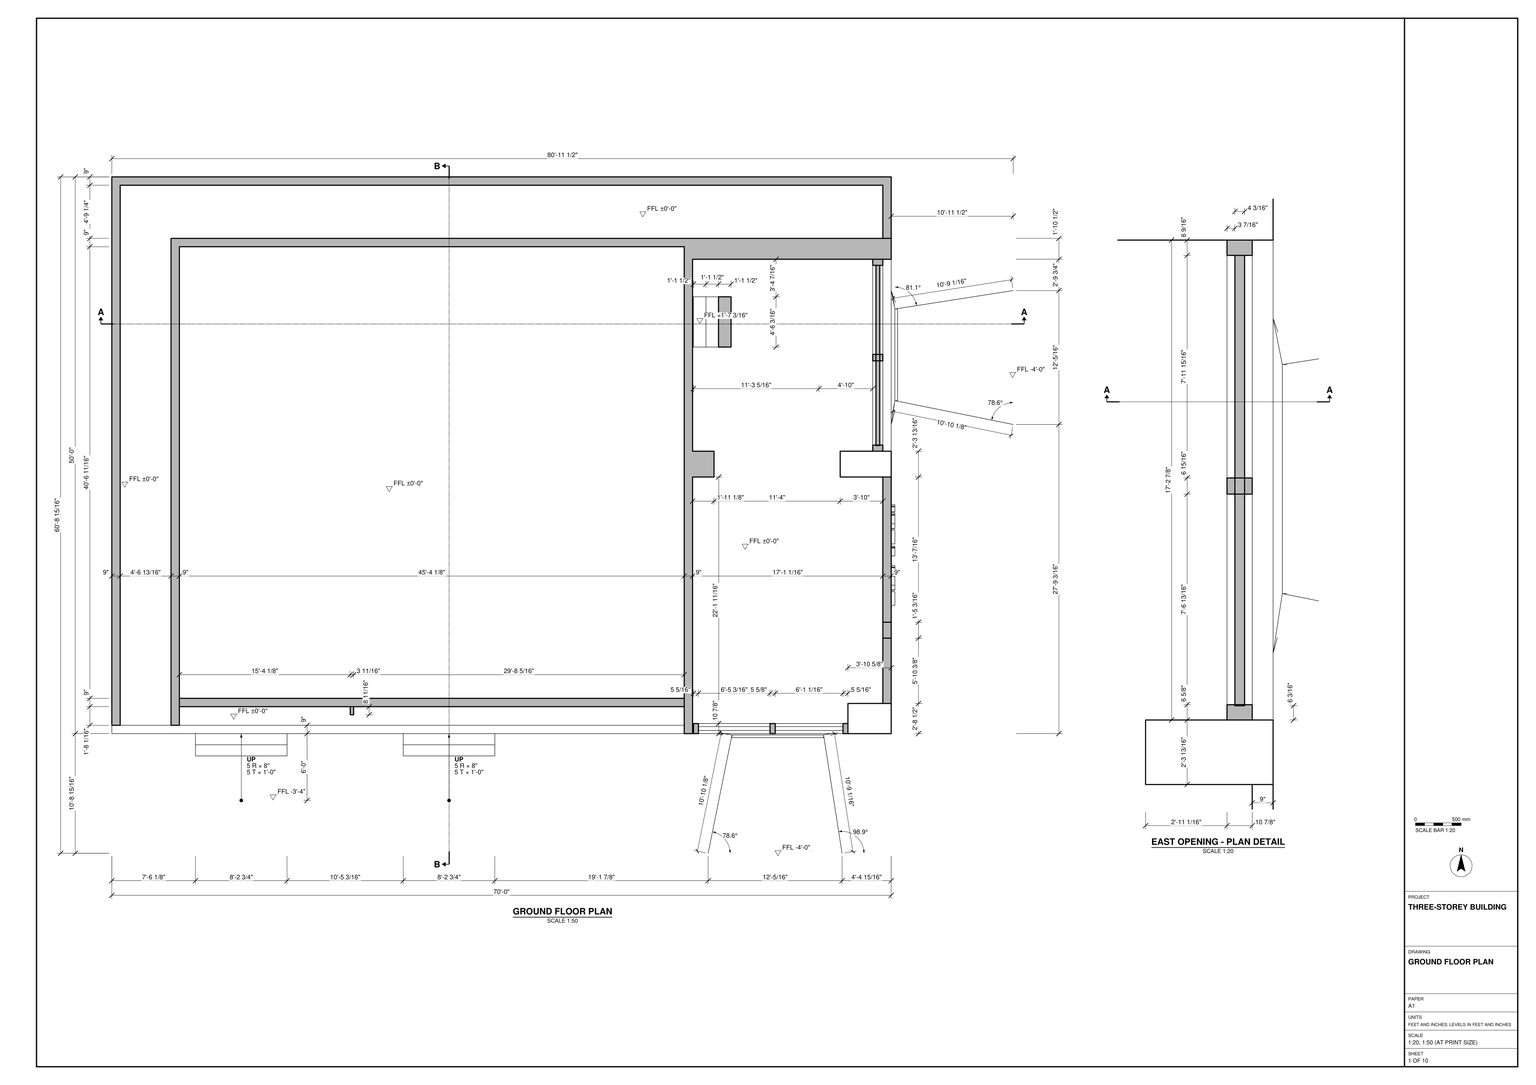
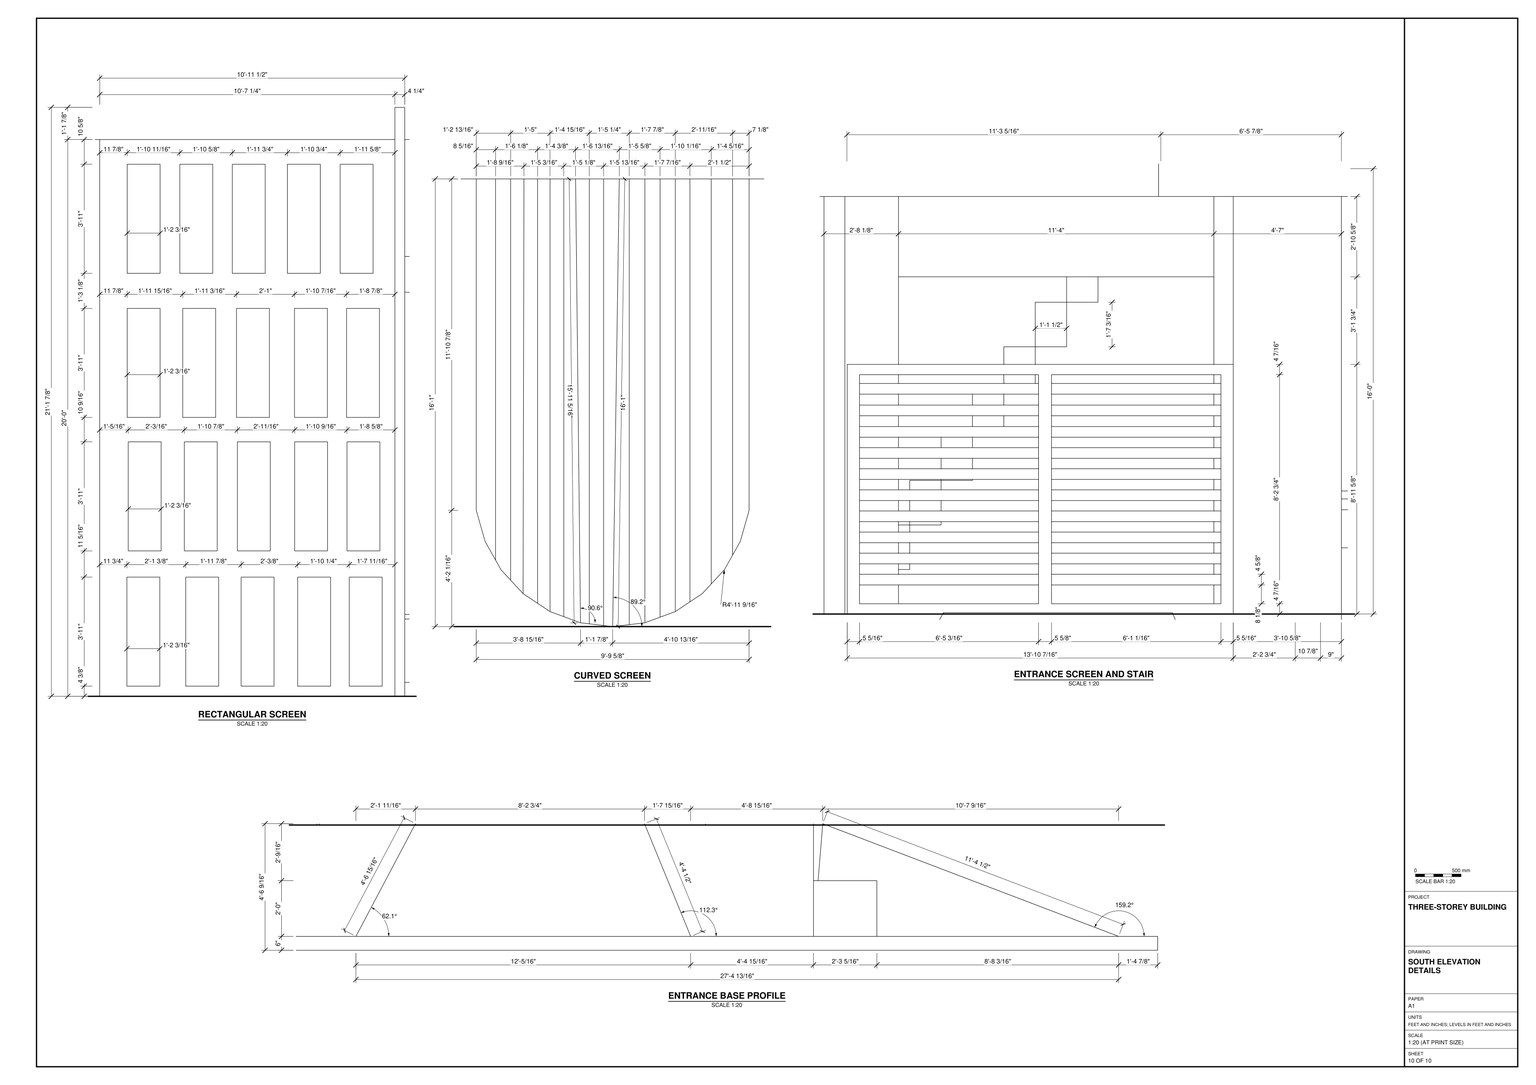
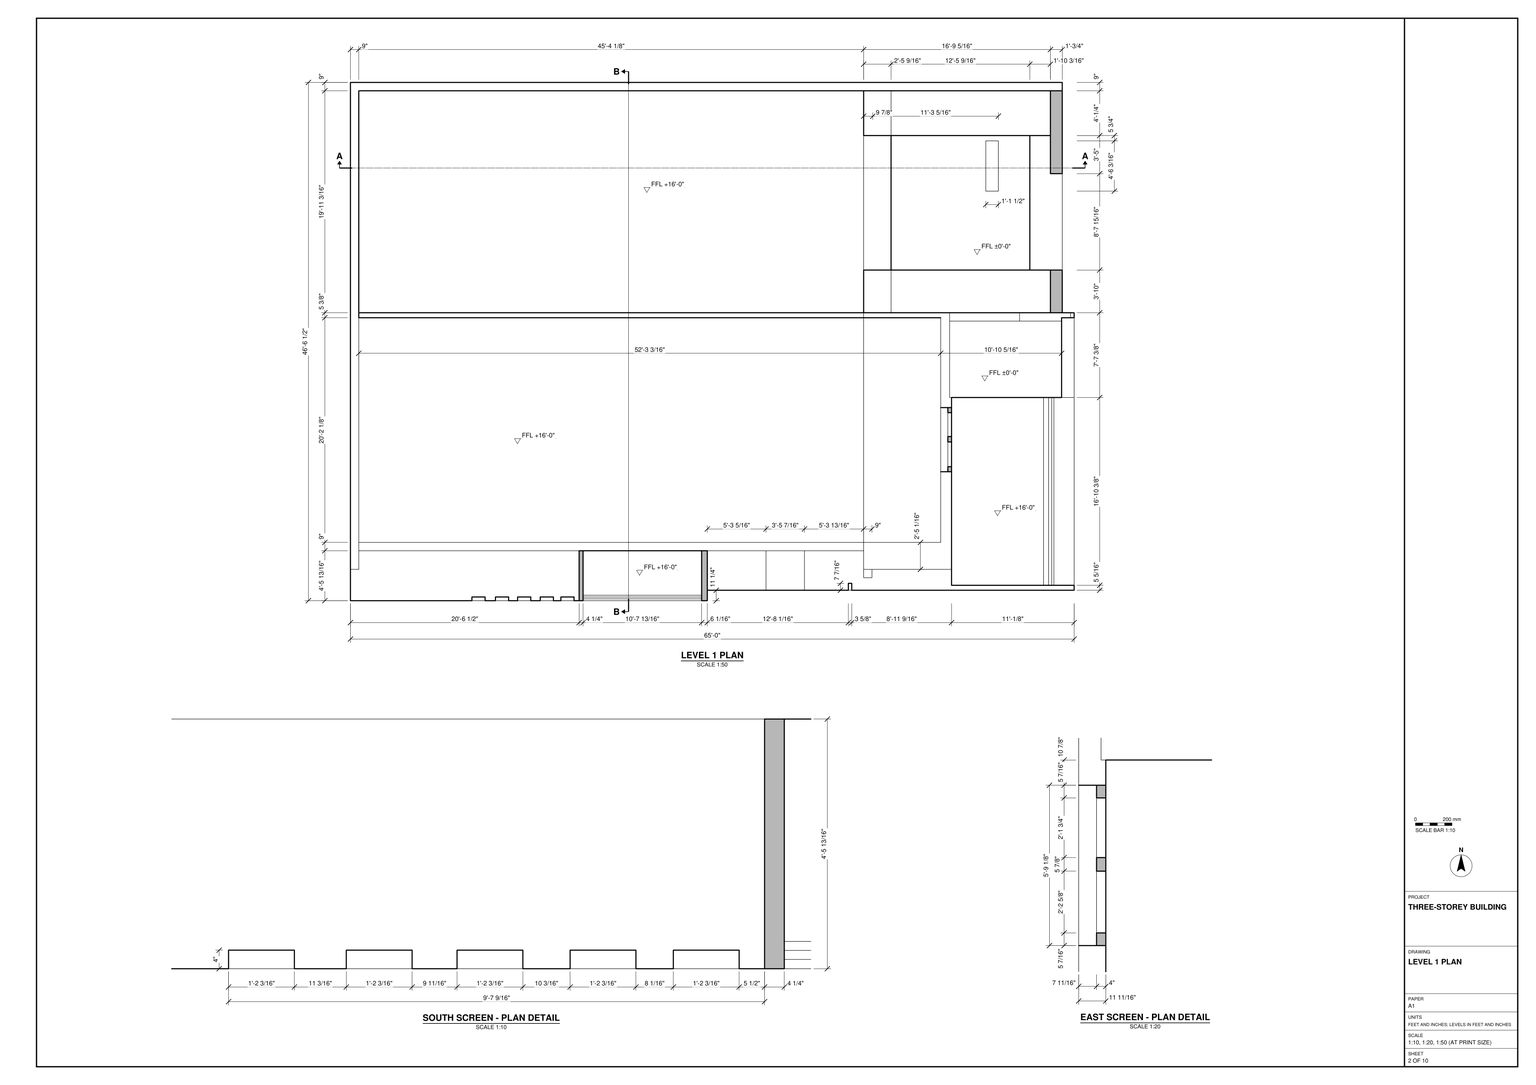
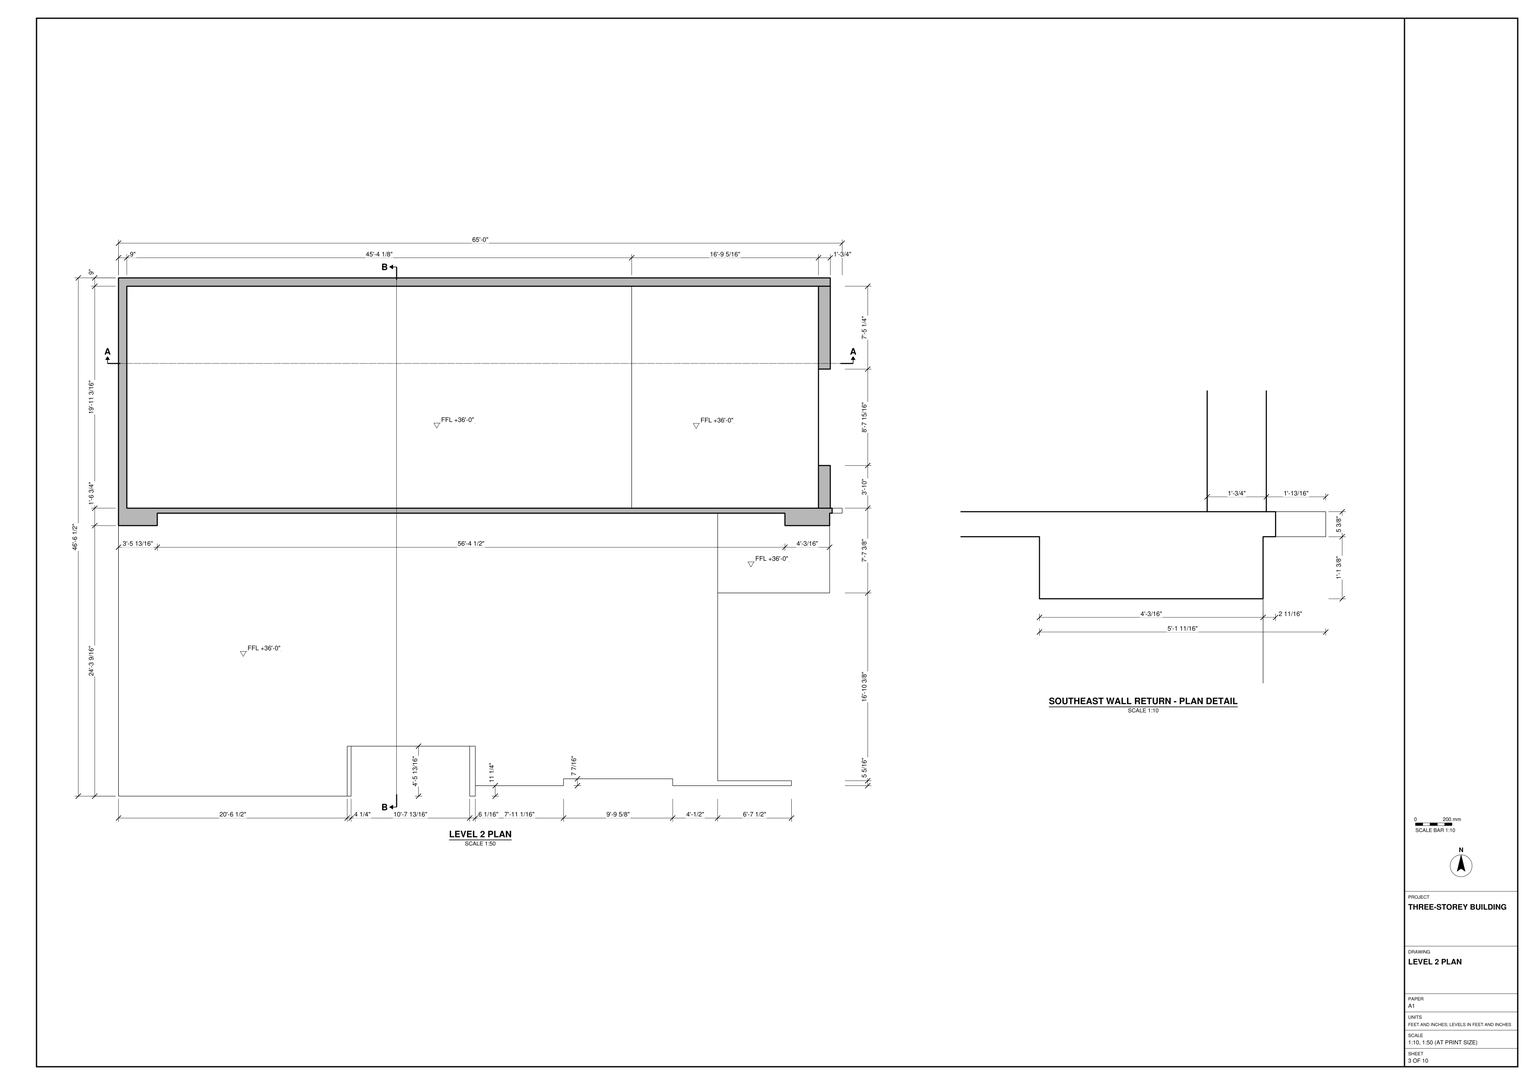
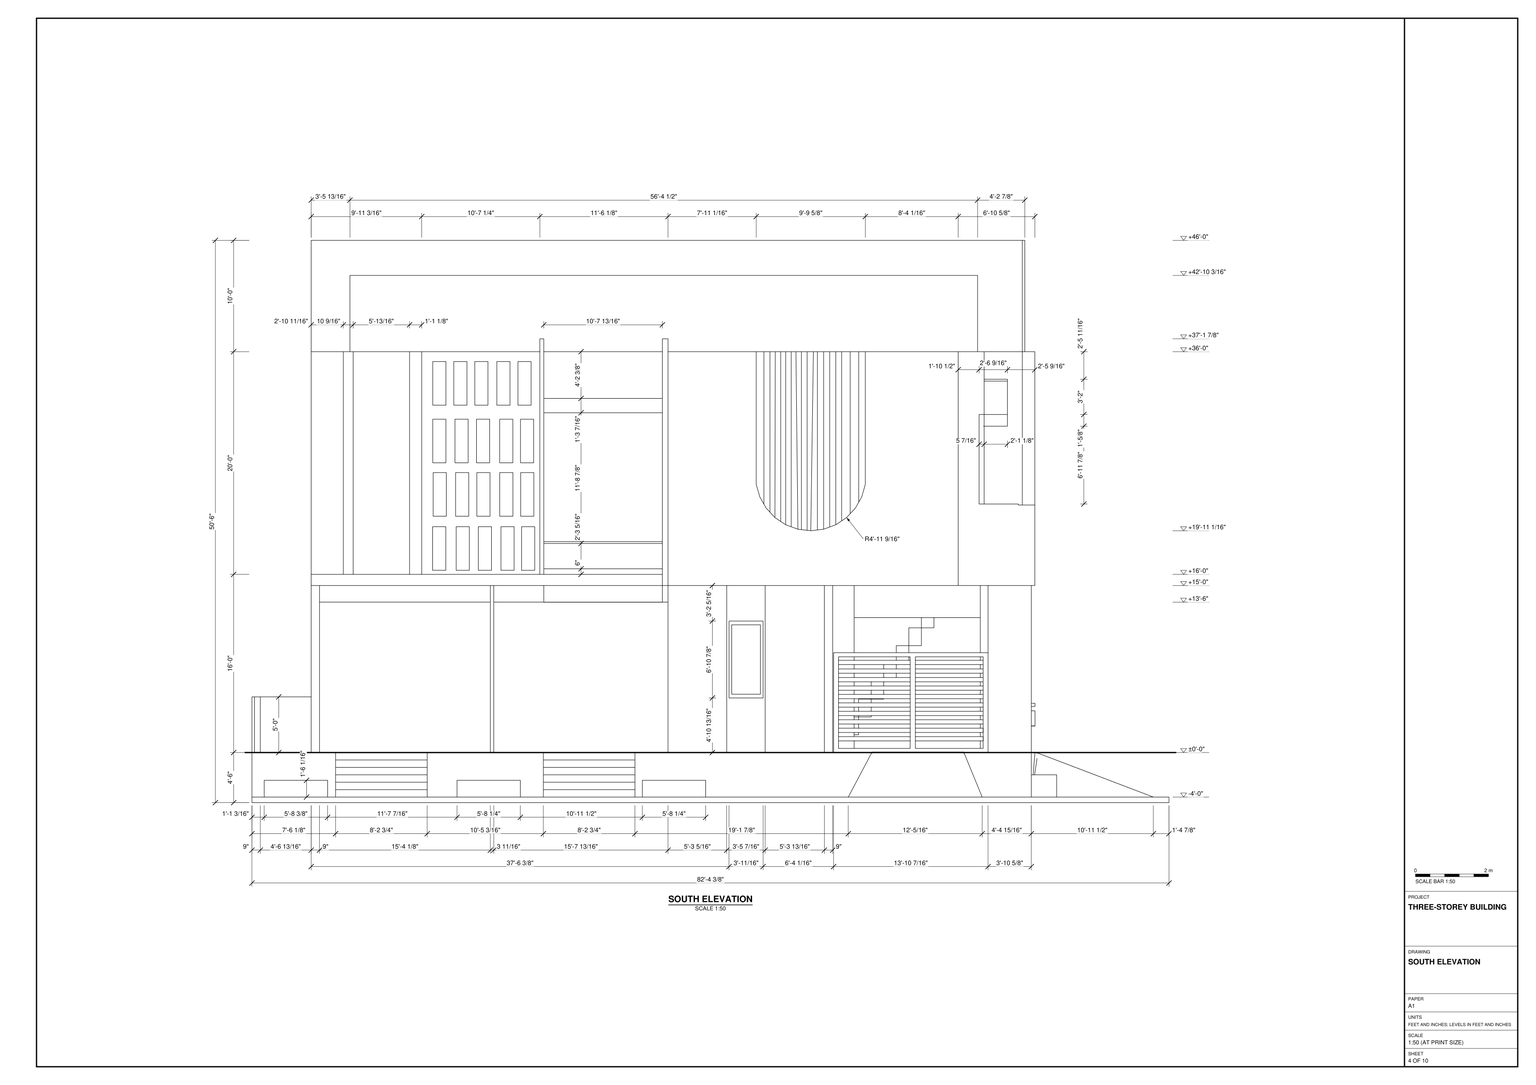
Use the plans, sections, elevations and details in task_files/diagram_01.pdf to build the three-storey building in SketchUp. Work in feet and inches. The complete model measures 82'-4 3/8" along X, 67'-10 1/8" along Y and 50'-6" along Z. Set the ground floor at ±0'-0" and the upper floors at +16'-0" and +36'-0".

Lay out the broad ground-floor space and the narrower east bay, using the wall thicknesses shown in plan. Model the floor slabs, openings, stairs and roof. Follow each floor plan rather than repeating the ground-floor outline: parts of the east bay remain open to the floor below. Include the two sets of south steps, the sloping entrance base and the framing of the east opening. Use the south elevation details to distinguish the rectangular grid screen, the vertical screen with a curved lower edge and the horizontal slats in front of the entrance stair.

Keep walls, slabs and roof as separate groups or components, and do the same for each furniture or built-in joinery piece shown. Use components for repeated parts. Any decor or loose items shown may use suitable library components. Save one SketchUp model as output_files/three_storey_building_with_facade_screens.skp.

# SketchUp Ruby script. Lengths in inches.
U = 1.inch
M = Sketchup.active_model
def pt(a) = Geom::Point3d.new(a.map { |v| v * U })
def face(e, loops, mat)
  f = e.add_face(loops[0].map { |a| pt(a) })
  loops[1..].each { |l| e.add_face(l.map { |a| pt(a) }).erase! }
  f.material = f.back_material = mat if mat
  f
end
# faces: each face lists its corners as indices into pts; further lists are holes
def faces(e, pts, list, mat = nil) = list.each { |f| face(e, (f[0].is_a?(Array) ? f : [f]).map { |l| l.map { |i| pts[i] } }, mat) }
# xy, xz, yz: faces in a plane at the given z, y or x. An outline is a flat list of corners, or four numbers for a rectangle; further outlines are holes
def ring(l) = l.size == 4 ? [[l[0], l[1]], [l[2], l[1]], [l[2], l[3]], [l[0], l[3]]] : l.each_slice(2).to_a
def flat(e, list, mat, &to3) = list.each { |f| face(e, (f[0].is_a?(Array) ? f : [f]).map { |l| ring(l).map { |u, v| to3.(u, v) } }, mat) }
def xy(e, z, list, mat = nil) = flat(e, list, mat) { |x, y| [x, y, z] }
def xz(e, y, list, mat = nil) = flat(e, list, mat) { |x, z| [x, y, z] }
def yz(e, x, list, mat = nil) = flat(e, list, mat) { |y, z| [x, y, z] }
def lines(e, pts, list) = list.each { |a, b| e.add_line(pt(pts[a]), pt(pts[b])) }
# prism: a flat outline (further loops are holes) pulled along v
def prism(e, loops, v, mat = nil)
  f = face(e, loops, mat); d = Geom::Vector3d.new(v.map { |x| x * U })
  f.pushpull(f.normal.samedirection?(d) ? d.length : -d.length)
end
def box(e, o, s, mat = nil) = prism(e, [[o, [o[0] + s[0], o[1], o[2]], [o[0] + s[0], o[1] + s[1], o[2]], [o[0], o[1] + s[1], o[2]]]], [0, 0, s[2]], mat)
def at(x, y, z, deg = 0) = Geom::Transformation.translation(pt([x, y, z])) * Geom::Transformation.rotation(ORIGIN, Z_AXIS, deg.degrees)
def axes(o, x, y, z) = Geom::Transformation.new([*x, 0, *y, 0, *z, 0, *pt(o).to_a, 1])
def part(name) = M.definitions.add(name)
# library, detail: a bought-in or finely detailed component or shape, given as its bounding box
def library(name, o, s) = part(name).tap { |d| box(d.entities, o, s) }
def detail(e, o, s) = box(e.add_group.entities, o, s)
def put(e, d, t, mat = nil) = e.add_instance(d, t).tap { |i| i.material = mat if mat }
def group(e, t, mat = nil) = e.add_group.tap { |g| g.transformation = t; g.material = mat if mat }.entities
root = M.entities
M.materials.add("[Blinds Roman Hobbled Blue]").color = [81, 82, 87]
M.materials.add("[Color C06]").color = [204, 102, 0]
M.materials.add("[Color C08]").color = [85, 51, 15]
M.materials.add("[Color D01]").color = [255, 242, 204]
M.materials.add("[Color M03]").color = [170, 170, 170]
M.materials.add("[Color M05]").color = [114, 114, 114]
M.materials.add("[Color M06]").color = [86, 86, 86]
M.materials.add("[Color M07]").color = [58, 58, 58]
M.materials.add("[Grass Dark Green]").color = [106, 157, 55]
M.materials.add("[Metal Seamed]").color = [118, 119, 115]
M.materials.add("[Rough Square Concrete Block]").color = [123, 120, 113]
M.materials.add("[Translucent Glass Blue]").color = [100, 149, 237]
M.materials["[Translucent Glass Blue]"].alpha = 0.5
M.materials.add("[Translucent Glass Gray]").color = [128, 128, 128]
M.materials["[Translucent Glass Gray]"].alpha = 0.5
c1 = library("om soni",[1.17,0,0],[108.57,24.51,4])
c2 = part("Group\#1")
xy(c2.entities,0,[[0,0,144.33,198.39]])
p = [[0,0,0],[144.33,0,0],[124.43,192.38,36.8],[25.68,192.38,36.8],[0,198.39,0],[144.33,198.39,0],
  [25.68,187.9375,35.5625],[124.43,187.9375,35.5625]]
faces(c2.entities,p,[[0,1,2,3],[0,3,4],[1,5,2],[4,6,7,5],[6,4,3],[7,2,5],[3,2,7,6]])
c3 = part("Group\#2")
box(c3.entities,[0,0,0],[20.5,54.1875,8])
c4 = library("Group\#4",[0,0,0],[166.4375,10.875,128.625])
c5 = part("Group\#5")
xy(c5.entities,0,[[0,0,18.6875,4]],"[Color C08]")
xy(c5.entities,1.47,[[1.47,0,8.67,4],[10.26,0,17.21,4]],"[Color C08]")
xy(c5.entities,28.76,[[1.47,0,8.67,4],[10.26,0,17.21,4]],"[Color C08]")
xy(c5.entities,30.24,[[0,0,18.6875,4]],"[Color C08]")
xz(c5.entities,0,[[[0,0,18.6875,30.24],[1.47,1.47,8.67,28.76],[10.26,1.47,17.21,28.76]]],"[Color C08]")
xz(c5.entities,0,[[1.47,1.47,8.67,28.76],[10.26,1.47,17.21,28.76]],"[Translucent Glass Gray]")
xz(c5.entities,4,[[[0,0,18.6875,30.24],[1.47,1.47,8.67,28.76],[10.26,1.47,17.21,28.76]]],"[Color C08]")
yz(c5.entities,0,[[0,0,4,30.24]],"[Color C08]")
yz(c5.entities,1.47,[[0,1.47,4,28.76]],"[Color C08]")
yz(c5.entities,8.67,[[0,1.47,4,28.76]],"[Color C08]")
yz(c5.entities,10.26,[[0,1.47,4,28.76]],"[Color C08]")
yz(c5.entities,17.21,[[0,1.47,4,28.76]],"[Color C08]")
yz(c5.entities,18.6875,[[0,0,4,30.24]],"[Color C08]")
xy(root,0,[[0,0,988.375,814.125]])
xy(root,6,[[90.14,142.125,188.89,154.125],[314.08,142.125,412.83,154.125],[90.14,154.125,188.89,214.125],[314.08,154.125,412.83,214.125],[0,214.125,0,814.125,840,814.125,840,521.03,867.3125,521.03,867.3125,334.22,840,334.22,840,214.125]])
xy(root,6,[[0,0,988.375,0,988.375,814.125,840,814.125,840,521.03,867.3125,521.03,867.3125,334.22,840,334.22,840,214.125,489.03,214.125,489.03,152.9375,420.78,152.9375,420.78,214.125,412.83,214.125,412.83,142.125,314.08,142.125,314.08,214.125,289.28,214.125,289.28,152.9375,221.03,152.9375,221.03,214.125,188.89,214.125,188.89,142.125,90.14,142.125,90.14,214.125,81.59,214.125,81.59,141.5625,13.22,141.5625,13.22,214.125,0,214.125]],"[Rough Square Concrete Block]")
xy(root,14,[[90.14,142.125,188.89,154.125],[314.08,142.125,412.83,154.125]])
xy(root,22,[[90.14,154.125,188.89,166.125],[314.08,154.125,412.83,166.125]])
xy(root,24.0625,[[13.22,141.5625,81.59,214.125],[221.03,152.9375,289.28,214.125],[420.78,152.9375,489.03,214.125]],"[Color C06]")
xy(root,30,[[90.14,166.125,188.89,178.125],[314.08,166.125,412.83,178.125]])
xy(root,30,[[840,334.22,867.3125,521.03]],"[Grass Dark Green]")
xy(root,38,[[90.14,178.125,188.89,190.125],[314.08,178.125,412.83,190.125]])
xy(root,46,[[90.14,190.125,188.89,202.125],[314.08,190.125,412.83,202.125]])
xy(root,54,[[90.14,202.125,188.89,214.125],[314.08,202.125,412.83,214.125],[0,214.125,616.9375,223.125],[616.9375,214.125,616.9375,738.875,72.8125,738.875,72.8125,223.125,63.8125,223.125,63.8125,747.875,840,747.875,840,725.375,625.9375,725.375,625.9375,518.5,649.05,518.5,649.05,490.6875,625.9375,490.6875,625.9375,214.125],[625.9375,214.125,793.375,223.125],
  [0,223.125,0,814.125,840,814.125,840,747.875,831,747.875,831,805.125,9,805.125,9,223.125],[9,223.125,63.8125,223.125,63.8125,747.875,831,747.875,831,805.125,9,805.125],[72.8125,223.125,616.9375,223.125,616.9375,243.1875,260.625,243.1875,260.625,234.5,256.96,234.5,256.96,243.1875,72.8125,243.1875],[625.9375,223.125,793.375,223.125,793.375,246.66,831,246.66,831,490.6875,785.03,490.6875,785.03,518.5,831,518.5,831,725.375,625.9375,725.375,625.9375,518.5,649.05,518.5,649.05,490.6875,625.9375,490.6875],[256.96,234.5,260.625,243.1875],
  [72.8125,243.1875,616.9375,252.1875],[72.8125,252.1875,616.9375,738.875],[831,334.22,840,490.6875],[785.03,490.6875,840,518.5],[831,518.5,840,725.375]])
xy(root,112.81,[[514.22,243.1875,550.9,252.1875]])
xy(root,114,[[0,223.125,9,223.125,9,805.125,831,805.125,831,747.875,840,747.875,840,814.125,0,814.125]])
xy(root,123.28,[[616.9375,358.22,625.9375,418.54]])
xy(root,126,[[831,334.22,840,412.45],[831,412.45,840,490.6875]])
xy(root,126,[[831,246.66,840,317.04]],"[Color C06]")
xy(root,130.125,[[831,317.04,840,334.22]],"[Color M06]")
xy(root,195.69,[[514.22,243.1875,550.9,252.1875]])
xy(root,196.78,[[616.9375,358.22,625.9375,418.54]])
xy(root,199.375,[[818.25,499.6875,826.05,518.5],[826.05,499.6875,831,518.5],[831,499.6875,840,518.5],[818.25,690.63,831,725.375],[831,725.375,840,747.875]])
xy(root,199.375,[[649.05,490.6875,785.03,499.6875],[818.25,518.5,831,545.69],[818.25,545.69,831,690.63]],"[Color M06]")
xy(root,216,[[314.53,193.32,442.35,195.26]])
xy(root,216.11,[[72.8125,223.125,256.96,243.1875],[260.625,223.125,448.43,243.1875]])
xy(root,234,[[63.8125,189.375,256.96,223.125],[256.96,189.375,260.625,234.5],[260.625,189.375,448.43,223.125],[448.43,200.625,511.74,243.1875],[511.74,200.625,553.15,243.1875],
  [553.15,200.625,553.15,243.1875,616.9375,243.1875,616.9375,214.125,625.9375,214.125,625.9375,490.6875,843.8125,490.6875,843.8125,200.625],[72.8125,223.125,256.96,243.1875],[260.625,223.125,448.43,243.1875],[256.96,234.5,260.625,243.1875],[72.8125,243.1875,616.9375,252.1875],
  [785.03,490.6875,840,499.6875],[840,490.6875,843.8125,499.6875],[646.5,499.6875,649.05,518.5],[785.03,499.6875,818.25,518.5],[625.9375,518.5,646.5,725.375],
  [646.5,725.375,818.25,738.875]])
xy(root,236.5,[[793.375,214.125,840,246.66]])
xy(root,242,[[72.8125,252.1875,616.9375,738.875]])
xy(root,244.1875,[[830.3,408.34,843.8125,494.3]],"[Color D01]")
xy(root,246,[[63.8125,189.375,63.8125,223.125,72.8125,223.125,72.8125,243.1875,310.29,243.1875,310.29,189.375],[310.29,189.375,314.53,243.1875],[314.53,191.375,442.35,195.26],[314.53,195.26,442.35,243.1875],[711.6875,205.9375,810.86,205.9375,810.86,408.34,711.6875,408.34,711.6875,397.46,700,397.46,700,328.34,711.6875,328.34],
  [810.86,205.9375,821.99,408.34],[821.99,205.9375,843.8125,408.34],[616.9375,223.125,616.9375,252.1875,700,252.1875,700,328.34,711.6875,328.34,711.6875,223.125],[72.8125,252.1875,616.9375,494.3],[616.9375,252.1875,700,494.3],
  [700,397.46,700,494.3,616.9375,494.3,616.9375,499.6875,709.625,499.6875,709.625,408.34,711.6875,408.34,711.6875,397.46],[72.8125,494.3,616.9375,499.6875],[72.8125,499.6875,616.9375,738.875],[616.9375,499.6875,646.5,545.69],[646.5,499.6875,818.25,545.69],
  [616.9375,545.69,646.5,690.63],[616.9375,690.63,646.5,738.875],[646.5,690.63,818.25,738.875],[818.25,690.63,831,738.875]])
xy(root,246,[[314.53,189.375,442.35,191.375],[796.0625,545.69,831,545.69,831,649.6,818.25,649.6,818.25,690.63,796.0625,690.63]],"[Color M06]")
xy(root,250.375,[[194.74,189.375,208.93,193.375],[220.12,189.375,234.31,193.375],[243.99,189.375,258.18,193.375],[268.37,189.375,282.56,193.375],[290.62,189.375,304.81,193.375]])
xy(root,252,[[314.53,191.375,442.35,193.32],[314.53,193.32,442.35,195.26]])
xy(root,255,[[810.86,205.9375,816.29,408.34],[816.29,205.9375,819.67,408.34]])
xy(root,255,[[819.67,205.9375,821.99,408.34]],"[Color M05]")
xy(root,279.3125,[[314.53,193.32,442.35,195.26]])
xy(root,281.3125,[[314.53,193.32,442.35,195.26]],"[Metal Seamed]")
xy(root,289.25,[[816.29,205.9375,819.67,408.34]])
xy(root,291.25,[[816.29,205.9375,819.67,408.34]],"[Color M07]")
xy(root,297.375,[[194.74,189.375,208.93,193.375],[220.12,189.375,234.31,193.375],[243.99,189.375,258.18,193.375],[268.37,189.375,282.56,193.375],[290.62,189.375,304.81,193.375]])
xy(root,308.69,[[195.32,189.375,209.51,193.375],[219.51,189.375,233.69,193.375],[242.38,189.375,256.57,193.375],[267.07,189.375,281.26,193.375],[289.63,189.375,303.82,193.375]])
xy(root,320.74,[[826.05,200.625,843.8125,202.125],[826.05,202.125,843.8125,205.9375]])
xy(root,321.8,[[783.69,200.625,789.14,200.625,789.14,205.9375],[783.69,200.625,789.14,205.9375,783.69,205.9375],[789.14,200.625,826.05,205.9375]])
xy(root,341.6875,[[646.5,545.69,796.0625,690.63]])
xy(root,355.69,[[195.32,189.375,209.51,193.375],[219.51,189.375,233.69,193.375],[242.38,189.375,256.57,193.375],[267.07,189.375,281.26,193.375],[289.63,189.375,303.82,193.375]])
xy(root,358.5,[[700,328.34,711.6875,397.46]])
xy(root,366.22,[[194.875,189.375,209.0625,193.375],[218.8125,189.375,233,193.375],[242,189.375,256.1875,193.375],[267,189.375,281.1875,193.375],[289.4375,189.375,303.625,193.375]])
xy(root,405.69,[[711.6875,205.9375,814.25,408.34]],"[Color M05]")
xy(root,413.22,[[194.875,189.375,209.0625,193.375],[218.8125,189.375,233,193.375],[242,189.375,256.1875,193.375],[267,189.375,281.1875,193.375],[289.4375,189.375,303.625,193.375]])
xy(root,418.3,[[783.69,200.625,789.14,205.9375,789.14,200.625],[709.625,205.9375,785,205.9375,785,211.01,810.58,211.01,810.58,408.34,709.625,408.34],[785,205.9375,785,211.01,810.58,211.01,810.58,408.34,814.25,408.34,814.25,205.9375]])
xy(root,419.75,[[616.9375,545.69,796.0625,690.63],[796.0625,545.69,818.25,690.63]])
xy(root,420.16,[[314.53,198.625,442.35,243.1875]])
xy(root,428.35,[[194.875,189.375,209.0625,193.375],[217.5625,189.375,231.75,193.375],[240.1875,189.375,254.375,193.375],[263.9375,189.375,278.125,193.375],[286.6875,189.375,300.875,193.375]])
xy(root,435.62,[[314.53,198.625,442.35,243.1875]],"[Grass Dark Green]")
xy(root,454.3,[[785,205.9375,785,211.01,810.58,211.01,810.58,408.34,814.25,408.34,814.25,205.9375]])
xy(root,456.3,[[785,205.9375,814.25,205.9375,814.25,408.34,810.58,408.34,810.58,211.01,785,211.01]],"[Color M07]")
xy(root,475.35,[[194.875,189.375,209.0625,193.375],[217.5625,189.375,231.75,193.375],[240.1875,189.375,254.375,193.375],[263.9375,189.375,278.125,193.375],[286.6875,189.375,300.875,193.375]])
xy(root,486,[[63.8125,189.375,310.29,189.375,310.29,243.1875,448.43,243.1875,448.43,200.625,543.48,200.625,543.48,208.0625,661.1,208.0625,661.1,200.625,789.14,200.625,789.14,205.9375,709.625,205.9375,709.625,494.3,105.6,494.3,105.6,480.92,63.8125,480.92],[72.8125,480.92,105.6,494.3],[782.1,480.92,782.1,494.3,72.8125,494.3,72.8125,499.6875,833,499.6875,833,494.3,830.3,494.3,830.3,480.92],[72.8125,499.6875,616.9375,738.875],[616.9375,499.6875,818.25,738.875]])
xy(root,486,[[709.625,408.34,830.3,408.34,830.3,480.92,782.1,480.92,782.1,494.3,709.625,494.3]],"[Color C06]")
xy(root,486,[[833,494.3,843.8125,499.6875]],"[Color D01]")
xy(root,499.875,[[310.29,189.375,314.53,243.1875],[442.35,189.375,448.43,243.1875]],"[Color M06]")
xy(root,549.25,[[818.25,545.69,831,649.6]],"[Color M06]")
xy(root,568.1875,[[105.6,480.92,782.1,494.3]],"[Color M05]")
xy(root,606,[[72.8125,499.6875,818.25,738.875]])
xy(root,606,[[63.8125,480.92,830.3,480.92,830.3,494.3,833,494.3,833,499.6875,72.8125,499.6875,72.8125,738.875,831,738.875,831,747.875,63.8125,747.875],[818.25,499.6875,831,738.875]],"[Color M05]")
xz(root,0,[[0,0,988.375,6]])
xz(root,141.5625,[[13.22,6,81.59,24.0625]],"[Color C06]")
xz(root,142.125,[[90.14,6,188.89,14],[314.08,6,412.83,14]])
xz(root,152.9375,[[221.03,6,289.28,24.0625],[420.78,6,489.03,24.0625]],"[Color C06]")
xz(root,154.125,[[90.14,14,188.89,22],[314.08,14,412.83,22]])
xz(root,166.125,[[90.14,22,188.89,30],[314.08,22,412.83,30]])
xz(root,178.125,[[90.14,30,188.89,38],[314.08,30,412.83,38]])
xz(root,189.375,[[63.8125,246,98.49,486],[109.07,246,169.87,486],[[183.02,246,310.29,486],[194.875,428.35,209.0625,475.35],[217.5625,428.35,231.75,475.35],[240.1875,428.35,254.375,475.35],[263.9375,428.35,278.125,475.35],[286.6875,428.35,300.875,475.35],[194.875,366.22,209.0625,413.22],[218.8125,366.22,233,413.22],[242,366.22,256.1875,413.22],[267,366.22,281.1875,413.22],[289.4375,366.22,303.625,413.22],[195.32,308.69,209.51,355.69],[219.51,308.69,233.69,355.69],[242.38,308.69,256.57,355.69],[267.07,308.69,281.26,355.69],[289.63,308.69,303.82,355.69],[194.74,250.375,208.93,297.375],[220.12,250.375,234.31,297.375],[243.99,250.375,258.18,297.375],[268.37,250.375,282.56,297.375],[290.62,250.375,304.81,297.375]]])
xz(root,189.375,[[63.8125,234,442.35,246],[442.35,234,448.43,499.875],[98.49,246,109.07,486],[169.87,246,183.02,486],[310.29,246,314.53,499.875]],"[Color M06]")
xz(root,190.125,[[90.14,38,188.89,46],[314.08,38,412.83,46]])
xz(root,191.375,[[314.53,246,442.35,252]])
xz(root,193.32,[[314.53,216,442.35,252]])
xz(root,193.32,[[314.53,279.3125,442.35,281.3125]],"[Metal Seamed]")
xz(root,193.32,[[314.53,252,442.35,279.3125]],"[Translucent Glass Blue]")
xz(root,193.375,[[194.74,250.375,208.93,297.375],[220.12,250.375,234.31,297.375],[243.99,250.375,258.18,297.375],[268.37,250.375,282.56,297.375],[290.62,250.375,304.81,297.375],
  [195.32,308.69,209.51,355.69],[219.51,308.69,233.69,355.69],[242.38,308.69,256.57,355.69],[267.07,308.69,281.26,355.69],[289.63,308.69,303.82,355.69],
  [194.875,366.22,209.0625,413.22],[218.8125,366.22,233,413.22],[242,366.22,256.1875,413.22],[267,366.22,281.1875,413.22],[289.4375,366.22,303.625,413.22],
  [194.875,428.35,209.0625,475.35],[217.5625,428.35,231.75,475.35],[240.1875,428.35,254.375,475.35],[263.9375,428.35,278.125,475.35],[286.6875,428.35,300.875,475.35]])
xz(root,195.26,[[314.53,216,442.35,246],[314.53,246,442.35,252]])
xz(root,195.26,[[314.53,279.3125,442.35,281.3125]],"[Metal Seamed]")
xz(root,195.26,[[314.53,252,442.35,279.3125]],"[Translucent Glass Blue]")
xz(root,198.625,[[314.53,420.16,442.35,435.62]])
xz(root,200.625,[[448.43,234,761.19,234,761.19,486,661.1,486,661.1,343.125,657.28,329.68,650.42,317.5,640.92,307.25,629.29,299.5,616.17,294.67,602.29,293.03,588.41,294.67,575.29,299.5,563.66,307.25,554.16,317.5,547.3,329.68,543.48,343.125,543.48,486,448.43,486],[761.19,234,843.8125,234,843.8125,320.74,826.05,320.74,826.05,321.8,783.69,321.8,783.69,418.3,789.14,418.3,789.14,486,761.19,486]])
xz(root,202.125,[[90.14,46,188.89,54],[314.08,46,412.83,54]])
xz(root,205.9375,[[711.6875,246,711.6875,405.69,789.14,405.69,789.14,321.8,783.69,321.8,783.69,320.74,843.8125,320.74,843.8125,246,821.99,246,821.99,255,819.67,255,819.67,291.25,816.29,291.25,816.29,255,810.86,255,810.86,246],[810.86,246,821.99,255],[816.29,255,819.67,289.25],[816.29,289.25,819.67,291.25],[783.69,320.74,789.14,321.8],
  [789.14,320.74,826.05,321.8],[709.625,418.3,709.625,486,789.14,486,789.14,456.3,785,456.3,785,418.3],[785,418.3,789.14,454.3],[785,454.3,789.14,456.3]])
xz(root,205.9375,[[789.14,405.69,814.25,418.3]],"[Color M05]")
xz(root,205.9375,[[789.14,454.3,814.25,456.3]],"[Color M07]")
xz(root,205.9375,[[789.14,418.3,814.25,454.3]],"[Translucent Glass Gray]")
xz(root,208.0625,[[602.29,293.03,605.13,486,598.375,486,598.375,293.49],[602.29,293.03,609.44,293.875,609.44,486,605.13,486],[598.375,293.49,598.375,486,592.21,486,592.21,294.22],[609.44,293.875,616.17,294.67,616.17,486,609.44,486],[592.21,294.22,592.21,486,586.3,486,588.41,294.67],
  [588.41,294.67,586.3,486,581.22,486,581.22,297.3125],[616.17,294.67,622.73,297.08,622.73,486,616.17,486],[622.73,297.08,629.29,299.5,629.29,486,622.73,486],[581.22,297.3125,581.22,486,575.29,486,575.29,299.5],[575.29,299.5,575.29,486,569.91,486,569.91,303.09],
  [629.29,299.5,635.59,303.7,635.59,486,629.29,486],[569.91,303.09,569.91,486,564.04,486,563.66,307.25],[635.59,303.7,640.92,307.25,644.79,311.43,644.79,486,635.59,486],[563.66,307.25,564.04,486,558.3,486,558.3,313.04],[644.79,311.43,650.42,317.5,653.99,323.85,653.99,486,644.79,486],
  [558.3,313.04,558.3,486,551.79,486,551.79,321.71,554.16,317.5],[551.79,321.71,551.79,486,543.48,486,543.48,343.125,547.3,329.68],[653.99,323.85,657.28,329.68,661.1,343.125,661.1,486,653.99,486]],"[Color C06]")
xz(root,211.01,[[785,454.3,810.58,456.3]],"[Color M07]")
xz(root,211.01,[[785,418.3,810.58,454.3]],"[Translucent Glass Gray]")
xz(root,214.125,[[0,6,13.22,6,13.22,24.0625,81.59,24.0625,81.59,6,90.14,6,90.14,54,0,54],[13.22,6,81.59,24.0625],[90.14,6,188.89,10.97],[188.89,6,221.03,6,221.03,24.0625,289.28,24.0625,289.28,6,314.08,6,314.08,54,188.89,54],[221.03,6,289.28,24.0625],
  [314.08,6,412.83,46],[420.78,6,489.03,24.0625],[90.14,10.97,188.89,46],[90.14,46,188.89,54],[314.08,46,412.83,54],
  [616.9375,54,625.9375,234]])
xz(root,214.125,[[412.83,6,420.78,6,420.78,24.0625,489.03,24.0625,489.03,6,840,6,840,236.5,793.375,236.5,793.375,54,412.83,54]],"[Color M06]")
xz(root,223.125,[[0,54,2.75,114],[2.75,54,9,114],[63.8125,54,72.8125,234],[72.8125,216.11,256.96,234],[260.625,216.11,448.43,234],
  [63.8125,234,72.8125,246]])
xz(root,234.5,[[256.96,54,260.625,234]])
xz(root,243.1875,[[256.96,54,260.625,234],[448.43,54,511.74,234],[553.15,54,616.9375,234],[72.8125,216.11,256.96,234],[260.625,216.11,448.43,234],
  [72.8125,234,448.43,246],[310.29,246,314.53,486],[442.35,246,448.43,486],[314.53,420.16,442.35,435.62],[314.53,435.62,442.35,486],
  [310.29,486,314.53,499.875],[442.35,486,448.43,499.875]])
xz(root,243.1875,[[72.8125,54,256.96,216.11],[260.625,54,448.43,216.11]],"[Blinds Roman Hobbled Blue]")
xz(root,243.1875,[[[511.74,54,553.15,234],[514.22,112.81,550.9,195.69]],[314.53,246,442.35,420.16]],"[Color M06]")
xz(root,246.66,[[831,54,840,126]])
xz(root,246.66,[[793.375,54,793.375,236.5,840,236.5,840,126,831,126,831,54]],"[Color M06]")
xz(root,252.1875,[[[72.8125,54,616.9375,234],[514.22,112.81,550.9,195.69]],[72.8125,234,616.9375,242],[72.8125,242,616.9375,246]])
xz(root,317.04,[[831,54,840,126]])
xz(root,317.04,[[831,126,840,130.125]],"[Color M06]")
xz(root,328.34,[[700,246,711.6875,358.5]])
xz(root,334.22,[[831,54,840,126],[831,126,840,130.125]])
xz(root,334.22,[[840,6,867.3125,30]],"[Color M06]")
xz(root,358.22,[[616.9375,123.28,625.9375,196.78]])
xz(root,397.46,[[700,246,711.6875,358.5]])
xz(root,408.34,[[830.3,244.1875,843.8125,246],[810.86,246,821.99,255],[816.29,255,819.67,289.25],[816.29,289.25,819.67,291.25],[810.58,418.3,814.25,454.3],
  [810.58,454.3,814.25,456.3]])
xz(root,408.34,[[711.6875,246,810.86,246,810.86,255,816.29,255,816.29,291.25,819.67,291.25,819.67,255,821.99,255,821.99,246,830.3,246,830.3,486,709.625,486,709.625,418.3,810.58,418.3,810.58,456.3,814.25,456.3,814.25,405.69,711.6875,405.69]],"[Color C06]")
xz(root,418.54,[[616.9375,123.28,625.9375,196.78]])
xz(root,480.92,[[63.8125,486,105.6,486,105.6,568.1875,782.1,568.1875,782.1,486,830.3,486,830.3,606,63.8125,606]],"[Color M05]")
xz(root,490.6875,[[831,54,840,126]])
xz(root,490.6875,[[625.9375,54,649.05,234],[785.03,54,831,54,831,126,840,126,840,234,785.03,234],[649.05,199.375,785.03,234]],"[Color M06]")
xz(root,494.3,[[72.8125,246,700,486],[830.3,486,833,606]])
xz(root,494.3,[[830.3,244.1875,843.8125,486]],"[Color D01]")
xz(root,494.3,[[105.6,486,782.1,568.1875]],"[Color M05]")
xz(root,499.6875,[[818.25,199.375,826.05,234],[826.05,199.375,831,234],[831,199.375,840,234],[831,234,843.8125,246],[72.8125,246,616.9375,486],
  [616.9375,246,818.25,486],[818.25,246,831,486],[72.8125,486,616.9375,606],[616.9375,486,818.25,606],[818.25,486,831,606],
  [831,486,833,606]])
xz(root,499.6875,[[831,246,843.8125,486]],"[Color D01]")
xz(root,499.6875,[[649.05,199.375,649.05,234,646.5,234,646.5,246,818.25,246,818.25,234,785.03,234,785.03,199.375]],"[Color M06]")
xz(root,518.5,[[625.9375,54,649.05,234],[785.03,54,785.03,234,818.25,234,818.25,199.375,840,199.375,840,54]],"[Color M06]")
xz(root,521.03,[[840,6,867.3125,30]],"[Color M06]")
xz(root,545.69,[[818.25,199.375,831,246],[616.9375,246,616.9375,419.75,796.0625,419.75,796.0625,341.6875,646.5,341.6875,646.5,246],[646.5,246,796.0625,341.6875]])
xz(root,545.69,[[796.0625,246,818.25,419.75],[818.25,246,831,549.25]],"[Color M06]")
xz(root,649.6,[[818.25,246,831,549.25]],"[Color M06]")
xz(root,690.63,[[818.25,199.375,831,246],[616.9375,246,646.5,246,646.5,341.6875,796.0625,341.6875,796.0625,419.75,616.9375,419.75],[646.5,246,796.0625,341.6875],[796.0625,246,818.25,419.75]])
xz(root,725.375,[[625.9375,54,840,54,840,199.375,818.25,199.375,818.25,234,625.9375,234]],"[Color M06]")
xz(root,738.875,[[72.8125,54,616.9375,234],[72.8125,234,616.9375,242],[646.5,234,818.25,246],[72.8125,242,616.9375,246],[72.8125,246,616.9375,486],
  [616.9375,246,818.25,486],[818.25,246,831,606],[72.8125,486,88.4375,606],[88.4375,486,616.9375,606],[616.9375,486,818.25,606]])
xz(root,747.875,[[63.8125,54,63.8125,234,831,234,831,199.375,840,199.375,840,114,831,114,831,54],[831,54,840,114],[63.8125,234,831,246],[63.8125,246,831,606]])
xz(root,805.125,[[9,54,831,114]])
xz(root,814.125,[[0,0,988.375,6],[0,6,840,54],[0,54,840,114]])
yz(root,0,[[0,0,814.125,6],[214.125,6,814.125,54],[223.125,54,814.125,114]])
yz(root,9,[[223.125,54,805.125,114]])
yz(root,13.22,[[141.5625,6,214.125,24.0625]],"[Color C06]")
yz(root,63.8125,[[223.125,54,747.875,234],[189.375,234,223.125,246],[223.125,234,747.875,246],[189.375,246,189.375,486,480.92,486,480.92,606,747.875,606,747.875,246]])
yz(root,72.8125,[[223.125,54,243.1875,216.11],[243.1875,54,252.1875,234],[252.1875,54,738.875,234],[223.125,216.11,243.1875,234],[223.125,234,243.1875,246],
  [243.1875,234,252.1875,246],[252.1875,234,738.875,242],[252.1875,242,738.875,246],[494.3,246,499.6875,486],[499.6875,246,738.875,486],
  [499.6875,486,738.875,606]])
yz(root,81.59,[[141.5625,6,214.125,24.0625]],"[Color C06]")
yz(root,90.14,[[142.125,6,142.125,14,154.125,14,154.125,22,166.125,22,166.125,30,178.125,30,178.125,38,190.125,38,190.125,46,202.125,46,202.125,54,214.125,54,214.125,6]])
yz(root,105.6,[[480.92,486,494.3,568.1875]],"[Color M05]")
yz(root,188.89,[[142.125,6,214.125,6,214.125,54,202.125,54,202.125,46,190.125,46,190.125,38,178.125,38,178.125,30,166.125,30,166.125,22,154.125,22,154.125,14,142.125,14]])
yz(root,194.74,[[189.375,250.375,193.375,297.375]])
yz(root,194.875,[[189.375,366.22,193.375,413.22],[189.375,428.35,193.375,475.35]])
yz(root,195.32,[[189.375,308.69,193.375,355.69]])
yz(root,208.93,[[189.375,250.375,193.375,297.375]])
yz(root,209.0625,[[189.375,366.22,193.375,413.22],[189.375,428.35,193.375,475.35]])
yz(root,209.51,[[189.375,308.69,193.375,355.69]])
yz(root,217.5625,[[189.375,428.35,193.375,475.35]])
yz(root,218.8125,[[189.375,366.22,193.375,413.22]])
yz(root,219.51,[[189.375,308.69,193.375,355.69]])
yz(root,220.12,[[189.375,250.375,193.375,297.375]])
yz(root,221.03,[[152.9375,6,214.125,24.0625]],"[Color C06]")
yz(root,231.75,[[189.375,428.35,193.375,475.35]])
yz(root,233,[[189.375,366.22,193.375,413.22]])
yz(root,233.69,[[189.375,308.69,193.375,355.69]])
yz(root,234.31,[[189.375,250.375,193.375,297.375]])
yz(root,240.1875,[[189.375,428.35,193.375,475.35]])
yz(root,242,[[189.375,366.22,193.375,413.22]])
yz(root,242.38,[[189.375,308.69,193.375,355.69]])
yz(root,243.99,[[189.375,250.375,193.375,297.375]])
yz(root,254.375,[[189.375,428.35,193.375,475.35]])
yz(root,256.1875,[[189.375,366.22,193.375,413.22]])
yz(root,256.57,[[189.375,308.69,193.375,355.69]])
yz(root,256.96,[[234.5,54,243.1875,216.11],[223.125,216.11,234.5,234],[234.5,216.11,243.1875,234]])
yz(root,258.18,[[189.375,250.375,193.375,297.375]])
yz(root,260.625,[[234.5,54,243.1875,216.11],[223.125,216.11,234.5,234],[234.5,216.11,243.1875,234]])
yz(root,263.9375,[[189.375,428.35,193.375,475.35]])
yz(root,267,[[189.375,366.22,193.375,413.22]])
yz(root,267.07,[[189.375,308.69,193.375,355.69]])
yz(root,268.37,[[189.375,250.375,193.375,297.375]])
yz(root,278.125,[[189.375,428.35,193.375,475.35]])
yz(root,281.1875,[[189.375,366.22,193.375,413.22]])
yz(root,281.26,[[189.375,308.69,193.375,355.69]])
yz(root,282.56,[[189.375,250.375,193.375,297.375]])
yz(root,286.6875,[[189.375,428.35,193.375,475.35]])
yz(root,289.28,[[152.9375,6,214.125,24.0625]],"[Color C06]")
yz(root,289.4375,[[189.375,366.22,193.375,413.22]])
yz(root,289.63,[[189.375,308.69,193.375,355.69]])
yz(root,290.62,[[189.375,250.375,193.375,297.375]])
yz(root,300.875,[[189.375,428.35,193.375,475.35]])
yz(root,303.625,[[189.375,366.22,193.375,413.22]])
yz(root,303.82,[[189.375,308.69,193.375,355.69]])
yz(root,304.81,[[189.375,250.375,193.375,297.375]])
yz(root,310.29,[[189.375,246,243.1875,486],[189.375,486,243.1875,499.875]])
yz(root,314.08,[[142.125,6,142.125,14,154.125,14,154.125,22,166.125,22,166.125,30,178.125,30,178.125,38,190.125,38,190.125,46,202.125,46,202.125,54,214.125,54,214.125,6]])
yz(root,314.53,[[193.32,216,195.26,246],[191.375,246,193.32,252],[193.32,246,195.26,252],[193.32,252,195.26,279.3125],[193.32,279.3125,195.26,281.3125],
  [198.625,420.16,243.1875,435.62]])
yz(root,314.53,[[189.375,246,191.375,246,191.375,252,193.32,252,193.32,281.3125,195.26,281.3125,195.26,246,243.1875,246,243.1875,420.16,198.625,420.16,198.625,435.62,243.1875,435.62,243.1875,499.875,189.375,499.875]],"[Color M06]")
yz(root,412.83,[[142.125,6,214.125,6,214.125,54,202.125,54,202.125,46,190.125,46,190.125,38,178.125,38,178.125,30,166.125,30,166.125,22,154.125,22,154.125,14,142.125,14]])
yz(root,420.78,[[152.9375,6,214.125,24.0625]],"[Color C06]")
yz(root,442.35,[[193.32,216,195.26,246],[191.375,246,193.32,252],[193.32,246,195.26,252],[193.32,252,195.26,279.3125],[193.32,279.3125,195.26,281.3125],
  [198.625,420.16,243.1875,435.62]])
yz(root,442.35,[[189.375,246,189.375,499.875,243.1875,499.875,243.1875,435.62,198.625,435.62,198.625,420.16,243.1875,420.16,243.1875,246,195.26,246,195.26,281.3125,193.32,281.3125,193.32,252,191.375,252,191.375,246]],"[Color M06]")
yz(root,448.43,[[223.125,216.11,243.1875,234],[200.625,234,243.1875,246],[200.625,246,243.1875,486],[200.625,486,243.1875,499.875]])
yz(root,448.43,[[189.375,234,200.625,499.875]],"[Color M06]")
yz(root,489.03,[[152.9375,6,214.125,24.0625]],"[Color C06]")
yz(root,514.22,[[243.1875,112.81,252.1875,195.69]])
yz(root,543.48,[[200.625,343.125,208.0625,486]],"[Color C06]")
yz(root,550.9,[[243.1875,112.81,252.1875,195.69]])
yz(root,616.9375,[[214.125,54,243.1875,234],[243.1875,54,252.1875,234],[[252.1875,54,738.875,234],[358.22,123.28,418.54,196.78]],[223.125,234,252.1875,246],[252.1875,234,738.875,242],
  [252.1875,242,494.3,246],[494.3,242,499.6875,246],[499.6875,242,545.69,246],[545.69,242,690.63,246],[690.63,242,714.75,246],
  [714.75,242,738.875,246],[499.6875,246,499.6875,486,738.875,486,738.875,246,690.63,246,690.63,419.75,545.69,419.75,545.69,246]])
yz(root,625.9375,[[[214.125,54,490.6875,234],[358.22,123.28,418.54,196.78]]],"[Color M03]")
yz(root,625.9375,[[518.5,54,725.375,234]],"[Color M06]")
yz(root,646.5,[[499.6875,234,738.875,246],[545.69,246,690.63,341.6875]])
yz(root,649.05,[[490.6875,199.375,499.6875,234]])
yz(root,649.05,[[490.6875,54,518.5,199.375],[499.6875,199.375,518.5,234]],"[Color M06]")
yz(root,661.1,[[200.625,343.125,208.0625,486]],"[Color C06]")
yz(root,709.625,[[205.9375,418.3,408.34,486]],"[Color M03]")
yz(root,711.6875,[[205.9375,246,328.34,246,328.34,358.5,397.46,358.5,397.46,246,408.34,246,408.34,405.69,205.9375,405.69]],"[Color M03]")
yz(root,782.1,[[480.92,486,494.3,568.1875]])
yz(root,785,[[205.9375,418.3,211.01,454.3],[205.9375,454.3,211.01,456.3]])
yz(root,785.03,[[490.6875,199.375,499.6875,234],[499.6875,199.375,518.5,234]])
yz(root,785.03,[[490.6875,54,518.5,199.375]],"[Color M06]")
yz(root,789.14,[[200.625,418.3,205.9375,486]])
yz(root,793.375,[[214.125,54,246.66,236.5]],"[Color M06]")
yz(root,796.0625,[[545.69,246,690.63,341.6875],[545.69,341.6875,690.63,419.75]],"[Color M06]")
yz(root,810.58,[[211.01,454.3,408.34,456.3]],"[Color M07]")
yz(root,810.58,[[211.01,418.3,408.34,454.3]],"[Translucent Glass Gray]")
yz(root,810.86,[[205.9375,246,408.34,255]])
yz(root,814.25,[[205.9375,405.69,408.34,418.3]],"[Color M05]")
yz(root,814.25,[[205.9375,418.3,207.35,454.3],[205.9375,454.3,207.35,456.3],[207.35,454.3,408.34,456.3]],"[Color M07]")
yz(root,814.25,[[207.35,418.3,408.34,454.3]],"[Translucent Glass Gray]")
yz(root,816.29,[[205.9375,289.25,408.34,291.25]],"[Color M07]")
yz(root,816.29,[[205.9375,255,408.34,289.25]],"[Translucent Glass Gray]")
yz(root,818.25,[[499.6875,199.375,518.5,234],[518.5,199.375,518.5,234,499.6875,234,499.6875,246,545.69,246,545.69,199.375],[690.63,199.375,690.63,246,738.875,246,738.875,234,725.375,234,725.375,199.375],[499.6875,246,545.69,486],[649.6,246,690.63,419.75],
  [690.63,246,738.875,246,738.875,486,649.6,486,649.6,419.75,690.63,419.75],[499.6875,486,499.6875,606,738.875,606,738.875,486,649.6,486,649.6,549.25,545.69,549.25,545.69,486]])
yz(root,818.25,[[545.69,419.75,649.6,486],[545.69,486,649.6,549.25]],"[Color M06]")
yz(root,819.67,[[205.9375,289.25,408.34,291.25]],"[Color M07]")
yz(root,819.67,[[205.9375,255,408.34,289.25]],"[Translucent Glass Gray]")
yz(root,821.99,[[205.9375,246,408.34,255]],"[Color M05]")
yz(root,826.05,[[200.625,320.74,202.125,321.8],[202.125,320.74,205.9375,321.8]])
yz(root,830.3,[[408.34,244.1875,412.48,486],[412.48,244.1875,417.1,486],[417.1,244.1875,421.73,486],[421.73,244.1875,426.35,486],[426.35,244.1875,430.98,486],
  [430.98,244.1875,435.6,486],[435.6,244.1875,440.23,486],[440.23,244.1875,444.85,486],[444.85,244.1875,449.48,486],[449.48,244.1875,454.1,486],
  [454.1,244.1875,458.73,486],[458.73,244.1875,463.35,486],[463.35,244.1875,467.98,486],[467.98,244.1875,472.6,486],[472.6,244.1875,477.23,486],
  [477.23,244.1875,481.85,486],[481.85,244.1875,486.48,486],[486.48,244.1875,491.1,486],[491.1,244.1875,494.3,486]],"[Color C06]")
yz(root,830.3,[[480.92,486,494.3,606]],"[Color D01]")
yz(root,831,[[317.04,54,334.22,126],[334.22,54,490.6875,126],[747.875,54,805.125,114],[317.04,126,334.22,130.125]])
yz(root,831,[[246.66,54,317.04,126],[649.6,199.375,690.63,225.66],[649.6,225.66,690.63,245.79],[649.6,245.79,690.63,264.91],[649.6,264.91,690.63,285.91],
  [649.6,285.91,690.63,306.29],[649.6,306.29,690.63,327.47],[649.6,327.47,690.63,347.66],[649.6,347.66,690.63,367.47],[649.6,367.47,690.63,384.85],
  [649.6,384.85,690.63,402.16],[649.6,402.16,690.63,419.75],[649.6,419.75,690.63,439.57],[649.6,439.57,690.63,458.44],[649.6,458.44,690.63,478.82],
  [649.6,478.82,690.63,500.57],[649.6,500.57,690.63,525.69],[649.6,525.69,690.63,549.25]],"[Color C06]")
yz(root,831,[[499.6875,199.375,545.69,199.375,545.69,549.25,499.6875,606],[690.63,199.375,747.875,199.375,747.875,606,738.875,606,738.875,246,690.63,246],[690.63,246,738.875,246,738.875,606,690.63,549.25],[545.69,549.25,690.63,549.25,738.875,606,499.6875,606]],"[Color D01]")
yz(root,831,[[545.69,199.375,649.6,246]],"[Color M06]")
yz(root,833,[[494.3,486,499.6875,606]],"[Color D01]")
yz(root,840,[[521.03,6,814.125,6,814.125,54,334.22,54,334.22,30,521.03,30],[747.875,54,814.125,114]])
yz(root,840,[[246.66,6,317.04,126],[334.22,82.55,490.6875,102.91]],"[Color C06]")
yz(root,840,[[334.22,54,412.45,82.55],[412.45,54,490.6875,82.55],[334.22,102.91,412.45,126],[412.45,102.91,490.6875,126]],"[Color D01]")
yz(root,840,[[214.125,6,246.66,236.5],[317.04,6,334.22,130.125],[490.6875,54,518.5,54,518.5,199.375,499.6875,199.375,499.6875,234,490.6875,234],[725.375,54,747.875,199.375]],"[Color M06]")
yz(root,843.8125,[[200.625,234,499.6875,234,499.6875,486,494.3,486,494.3,244.1875,408.34,244.1875,408.34,246,205.9375,246,205.9375,320.74,200.625,320.74]],"[Color D01]")
yz(root,867.3125,[[334.22,6,521.03,30]],"[Color M06]")
yz(root,988.375,[[0,0,814.125,6]])
# 15 loose lines left out
p = [[588.41,200.625,294.67],[602.29,200.625,293.03],[602.29,208.0625,293.03],[598.375,208.0625,293.49],[592.21,208.0625,294.22],[588.41,208.0625,294.67],
  [616.17,200.625,294.67],[616.17,208.0625,294.67],[609.44,208.0625,293.875],[575.29,200.625,299.5],[581.22,208.0625,297.3125],[575.29,208.0625,299.5],
  [629.29,200.625,299.5],[629.29,208.0625,299.5],[622.73,208.0625,297.08],[563.66,200.625,307.25],[569.91,208.0625,303.09],[563.66,208.0625,307.25],
  [640.92,200.625,307.25],[640.92,208.0625,307.25],[635.59,208.0625,303.7],[554.16,200.625,317.5],[558.3,208.0625,313.04],[554.16,208.0625,317.5],
  [650.42,200.625,317.5],[650.42,208.0625,317.5],[644.79,208.0625,311.43],[547.3,200.625,329.68],[551.79,208.0625,321.71],[547.3,208.0625,329.68],
  [657.28,200.625,329.68],[657.28,208.0625,329.68],[653.99,208.0625,323.85],[783.69,200.625,418.3],[783.69,200.625,321.8],[789.14,205.9375,321.8],
  [789.14,205.9375,405.69],[789.14,205.9375,418.3],[543.48,200.625,343.125],[543.48,208.0625,343.125],[661.1,200.625,343.125],[661.1,208.0625,343.125]]
faces(root,p,[[0,1,2,3,4,5],[1,6,7,8,2],[9,0,5,10,11],[6,12,13,14,7],[15,9,11,16,17],[12,18,19,20,13],[21,15,17,22,23],[18,24,25,26,19],
  [27,21,23,28,29],[24,30,31,32,25],[38,27,29,39],[30,40,41,31]],"[Color C06]")
faces(root,p,[[33,34,35,36,37]])
put(root,c1,axes([840,351.08,82.55],[0,1,0],[0,0,1],[1,0,0]))
put(root,c2,axes([642.71,85.17,6],[1,0,0],[0,0.663,0],[0,0,1.32]))
g1 = group(root,at(762.13,684.91,54))
put(g1,c3,axes([-121.77,0,0],[-0.66,0,0],[0,-1,0],[0,0,2.4]))
put(g1,c3,axes([-27.06,0,134.4],[-0.66,0,0],[0,-1,0],[0,0,2.4]))
put(g1,c3,axes([0,0,172.8],[-0.66,0,0],[0,-1,0],[0,0,2.4]))
put(g1,c3,axes([-108.24,0,19.2],[-0.66,0,0],[0,-1,0],[0,0,2.4]))
put(g1,c3,axes([-94.71,0,38.4],[-0.66,0,0],[0,-1,0],[0,0,2.4]))
put(g1,c3,axes([-54.12,0,96],[-0.66,0,0],[0,-1,0],[0,0,2.4]))
put(g1,c3,axes([-67.65,0,76.8],[-0.66,0,0],[0,-1,0],[0,0,2.4]))
put(g1,c3,axes([-40.59,0,115.2],[-0.66,0,0],[0,-1,0],[0,0,2.4]))
put(g1,c3,axes([-81.18,0,57.6],[-0.66,0,0],[0,-1,0],[0,0,2.4]))
put(g1,c3,axes([-13.53,0,153.6],[-0.66,0,0],[0,-1,0],[0,0,2.4]))
put(root,c4,axes([626.9375,214.125,54],[1,0,0],[0,1,0],[0,0,0.8366]))
put(root,c4,axes([820.125,725.375,54],[0,-1.24296,0],[1,0,0],[0,0,0.75294]))
put(root,c2,axes([971.53,547.3125,6],[0,1,0],[-0.663,0,0],[0,0,1.32]))
put(root,c5,axes([625.4375,358.22,123.28],[0,3.22742,0],[-1,0,0],[0,0,2.4308]))
g2 = group(root,at(514.22,243.1875,112.81))
xy(g2,0,[[0,0,36.6875,4]],"[Color C08]")
xy(g2,4.04,[[2.9,0,33.79,4]],"[Color C08]")
xy(g2,78.83,[[2.9,0,33.79,4]],"[Color C08]")
xy(g2,82.875,[[0,0,36.6875,4]],"[Color C08]")
xz(g2,0,[[[0,0,36.6875,82.875],[2.9,4.04,33.79,78.83]]],"[Color C08]")
xz(g2,0,[[2.9,4.04,33.79,78.83]],"[Translucent Glass Gray]")
xz(g2,4,[[[0,0,36.6875,82.875],[2.9,4.04,33.79,78.83]]],"[Color C08]")
yz(g2,0,[[0,0,4,82.875]],"[Color C08]")
yz(g2,2.9,[[0,4.04,4,78.83]],"[Color C08]")
yz(g2,33.79,[[0,4.04,4,78.83]],"[Color C08]")
yz(g2,36.6875,[[0,0,4,82.875]],"[Color C08]")
put(root,c5,axes([711.6875,328.34,246],[0,3.699,0],[-1,0,0],[0,0,3.72061]))
